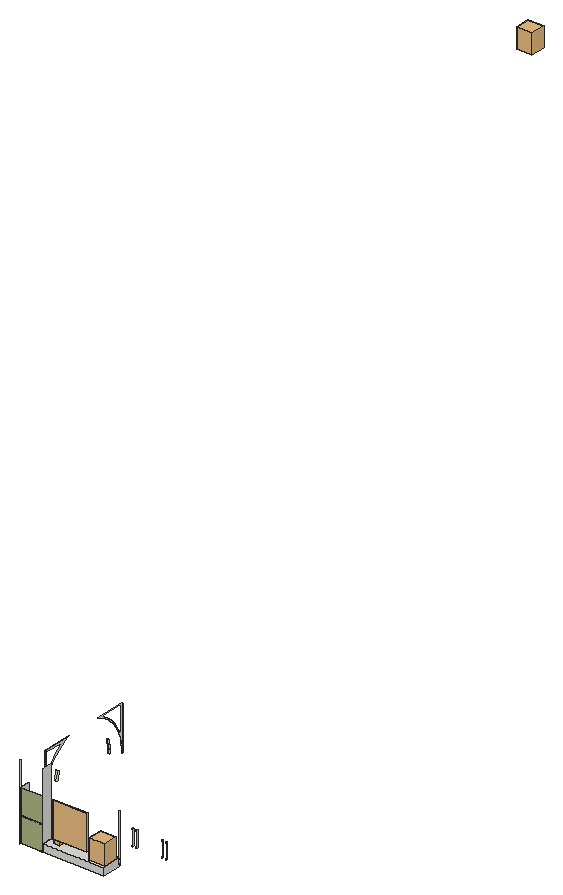
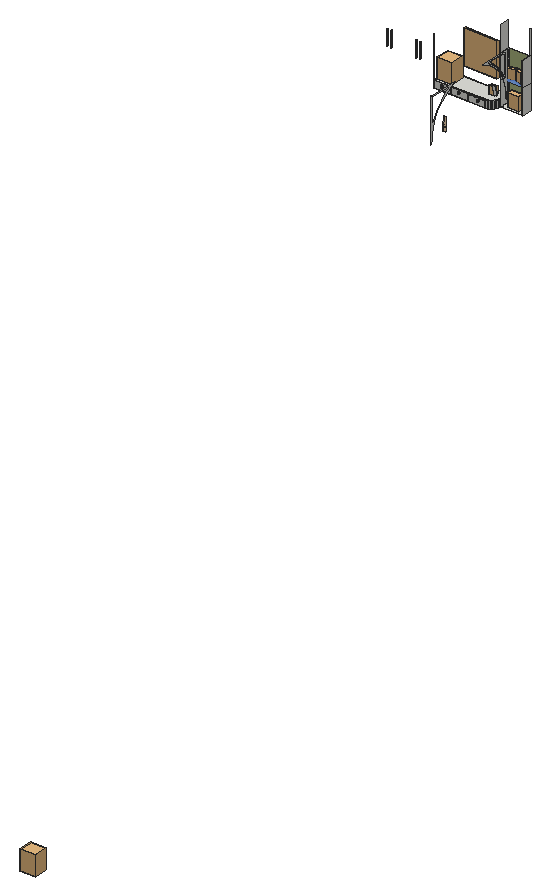
# SketchUp Ruby script. Lengths in inches.
U = 1.inch
M = Sketchup.active_model
def pt(a) = Geom::Point3d.new(a.map { |v| v * U })
def face(e, loops, mat)
  f = e.add_face(loops[0].map { |a| pt(a) })
  loops[1..].each { |l| e.add_face(l.map { |a| pt(a) }).erase! }
  f.material = f.back_material = mat if mat
  f
end
# faces: each face lists its corners as indices into pts; further lists are holes
def faces(e, pts, list, mat = nil) = list.each { |f| face(e, (f[0].is_a?(Array) ? f : [f]).map { |l| l.map { |i| pts[i] } }, mat) }
# xy, xz, yz: faces in a plane at the given z, y or x. An outline is a flat list of corners, or four numbers for a rectangle; further outlines are holes
def ring(l) = l.size == 4 ? [[l[0], l[1]], [l[2], l[1]], [l[2], l[3]], [l[0], l[3]]] : l.each_slice(2).to_a
def flat(e, list, mat, &to3) = list.each { |f| face(e, (f[0].is_a?(Array) ? f : [f]).map { |l| ring(l).map { |u, v| to3.(u, v) } }, mat) }
def xy(e, z, list, mat = nil) = flat(e, list, mat) { |x, y| [x, y, z] }
def xz(e, y, list, mat = nil) = flat(e, list, mat) { |x, z| [x, y, z] }
def yz(e, x, list, mat = nil) = flat(e, list, mat) { |y, z| [x, y, z] }
def lines(e, pts, list) = list.each { |a, b| e.add_line(pt(pts[a]), pt(pts[b])) }
# prism: a flat outline (further loops are holes) pulled along v
def prism(e, loops, v, mat = nil)
  f = face(e, loops, mat); d = Geom::Vector3d.new(v.map { |x| x * U })
  f.pushpull(f.normal.samedirection?(d) ? d.length : -d.length)
end
def box(e, o, s, mat = nil) = prism(e, [[o, [o[0] + s[0], o[1], o[2]], [o[0] + s[0], o[1] + s[1], o[2]], [o[0], o[1] + s[1], o[2]]]], [0, 0, s[2]], mat)
def at(x, y, z, deg = 0) = Geom::Transformation.translation(pt([x, y, z])) * Geom::Transformation.rotation(ORIGIN, Z_AXIS, deg.degrees)
def axes(o, x, y, z) = Geom::Transformation.new([*x, 0, *y, 0, *z, 0, *pt(o).to_a, 1])
def part(name) = M.definitions.add(name)
# library, detail: a bought-in or finely detailed component or shape, given as its bounding box
def library(name, o, s) = part(name).tap { |d| box(d.entities, o, s) }
def detail(e, o, s) = box(e.add_group.entities, o, s)
def put(e, d, t, mat = nil) = e.add_instance(d, t).tap { |i| i.material = mat if mat }
def group(e, t, mat = nil) = e.add_group.tap { |g| g.transformation = t; g.material = mat if mat }.entities
root = M.entities
M.materials.add("Emissive").color = [255, 225, 187]
M.materials.add("[Translucent Glass Blue]").color = [100, 149, 237]
M.materials["[Translucent Glass Blue]"].alpha = 0.5
M.materials.add("cubod").color = [174, 185, 130]
c1 = library("POTICHES",[0,0,0],[13.49,6.56,16.28])
c2 = part("Group\#11")
xz(c2.entities,1.09,[[1.15,0,0.85,0.04,0.57,0.15,0.34,0.33,0.15,0.56,0.04,0.83,0,1.12,0.04,1.41,0.15,1.68,0.34,1.91,0.57,2.09,0.85,2.2,1.15,2.24,1.45,2.2,1.72,2.09,1.96,1.91,2.14,1.68,2.26,1.41,2.3,1.12,2.26,0.83,2.14,0.56,1.96,0.33,1.72,0.15,1.45,0.04]])
p = [[0.57,1.09,0.15],[0.85,1.09,0.04],[0.85,0.7,0.04],[0.57,0.7,0.15],[1.15,1.09,0],[1.15,0.7,0],
  [1.45,1.09,0.04],[1.45,0.7,0.04],[1.72,1.09,0.15],[1.72,0.7,0.15],[0.34,1.09,0.33],[0.34,0.7,0.33],
  [1.96,1.09,0.33],[1.96,0.7,0.33],[0.15,1.09,0.56],[0.15,0.7,0.56],[2.14,1.09,0.56],[2.14,0.7,0.56],
  [1.02,0.7,0.65],[1.15,0.7,0.64],[1.15,0,0.64],[1.02,0,0.65],[1.28,0.7,0.65],[1.28,0,0.65],
  [0.04,1.09,0.83],[0.04,0.7,0.83],[2.26,1.09,0.83],[2.26,0.7,0.83],[0.8,0.7,0.78],[0.9,0.7,0.7],
  [0.9,0,0.7],[0.8,0,0.78],[1.4,0.7,0.7],[1.4,0,0.7],[1.5,0.7,0.78],[1.5,0,0.78],
  [0.72,0.7,0.88],[0.72,0,0.88],[1.58,0.7,0.88],[1.58,0,0.88],[0,1.09,1.12],[0,0.7,1.12],
  [2.3,1.09,1.12],[2.3,0.7,1.12],[0.67,0.7,0.99],[0.67,0,0.99],[1.63,0.7,0.99],[1.63,0,0.99],
  [0.65,0.7,1.12],[0.65,0,1.12],[1.65,0.7,1.12],[1.65,0,1.12],[0.67,0.7,1.25],[0.67,0,1.25],
  [1.63,0.7,1.25],[1.63,0,1.25],[0.04,1.09,1.41],[0.04,0.7,1.41],[2.26,1.09,1.41],[2.26,0.7,1.41],
  [0.72,0.7,1.36],[0.72,0,1.36],[1.58,0.7,1.36],[1.58,0,1.36],[0.8,0.7,1.46],[0.8,0,1.46],
  [1.5,0.7,1.46],[1.5,0,1.46],[0.15,1.09,1.68],[0.15,0.7,1.68],[2.14,1.09,1.68],[2.14,0.7,1.68],
  [0.9,0.7,1.54],[0.9,0,1.54],[1.02,0.7,1.59],[1.02,0,1.59],[1.4,0.7,1.54],[1.28,0.7,1.59],
  [1.28,0,1.59],[1.4,0,1.54],[1.15,0.7,1.6],[1.15,0,1.6],[0.34,1.09,1.91],[0.34,0.7,1.91],
  [1.96,1.09,1.91],[1.96,0.7,1.91],[0.57,1.09,2.09],[0.57,0.7,2.09],[1.72,1.09,2.09],[1.72,0.7,2.09],
  [0.85,1.09,2.2],[0.85,0.7,2.2],[1.45,1.09,2.2],[1.45,0.7,2.2],[1.15,1.09,2.24],[1.15,0.7,2.24]]
faces(c2.entities,p,[[0,1,2,3],[1,4,5,2],[4,6,7,5],[6,8,9,7],[10,0,3,11],[8,12,13,9],[14,10,11,15],[12,16,17,13],
  [18,19,20,21],[19,22,23,20],[24,14,15,25],[16,26,27,17],[28,29,30,31],[29,18,21,30],[22,32,33,23],[32,34,35,33],
  [36,28,31,37],[34,38,39,35],[40,24,25,41],[26,42,43,27],[44,36,37,45],[38,46,47,39],[48,44,45,49],[46,50,51,47],
  [52,48,49,53],[50,54,55,51],[56,40,41,57],[42,58,59,43],[60,52,53,61],[54,62,63,55],[64,60,61,65],[62,66,67,63],
  [68,56,57,69],[58,70,71,59],[72,64,65,73],[74,72,73,75],[76,77,78,79],[66,76,79,67],[80,74,75,81],[77,80,81,78],
  [82,68,69,83],[70,84,85,71],[86,82,83,87],[84,88,89,85],[90,86,87,91],[88,92,93,89],[94,90,91,95],[92,94,95,93]])
c3 = library("Vase with branches",[15.48,-1.66,0],[18.51,16.76,23.67])
c4 = library("Decor Livro e Telescópio",[-0.65,0.19,2.02],[7.35,4.61,9.12])
c5 = part("Group\#10")
prism(c5.entities,[[[1.125,0,43.59],[1.125,0,42.2],[1.125,4.02,42.2],[1.125,4.02,1.84],[1.125,3.28,1.84],[1.125,0,1.84],[1.125,0,0],[1.125,4.41,0],[1.125,4.53,0.01],[1.125,4.64,0.03],[1.125,4.76,0.07],[1.125,4.86,0.12],[1.125,4.96,0.1875],[1.125,5.05,0.26],[1.125,5.125,0.35],[1.125,5.19,0.45],[1.125,5.24,0.56],[1.125,5.28,0.67],[1.125,5.3,0.79],[1.125,5.3125,0.9],[1.125,5.3125,42.39],[1.125,5.3,42.54],[1.125,5.28,42.68],[1.125,5.23,42.82],[1.125,5.17,42.95],[1.125,5.1,43.08],[1.125,5,43.19],[1.125,4.9,43.3],[1.125,4.78,43.39],[1.125,4.66,43.46],[1.125,4.52,43.52],[1.125,4.38,43.56],[1.125,4.24,43.59]]],[-0.5625,0,0])
c6 = library("Agrupar\#9",[-3.82,0,-0.04],[36.26,88.57,114.21])
c7 = library("Agrupar\#8",[-3.82,0,-0.04],[36.26,88.57,114.21])
xy(root,34.31,[[616.04,4,616.04,16,616.12,17.36,616.35,18.7,616.73,20.01,617.25,21.26,617.92,22.45,618.71,23.56,619.63,24.5625,620.65,25.46,621.77,26.24,622.97,26.88,623.25,27,688.79,27,688.79,4]])
xy(root,34.39,[[589.4375,4,613.52,4.375],[613.52,4,615.39,4.375],[589.4375,4.375,615.39,16]])
xy(root,34.81,[[623.25,27,624.23,27.39,625.54,27.75,646.47,27.75,646.47,27.0625,646.625,27.0625,646.625,27.75,667.55,27.75,667.55,27.0625,667.71,27.0625,667.71,27.75,688.79,27.75,688.79,27]])
xy(root,42.88,[[623.25,27,688.79,27,688.79,27.75,667.71,27.75,667.71,27.0625,667.55,27.0625,667.55,27.75,646.625,27.75,646.625,27.0625,646.47,27.0625,646.47,27.75,625.54,27.75,624.23,27.39]])
xy(root,43.44,[[616.04,4,688.79,4,688.79,27,623.25,27,622.97,26.88,621.77,26.24,620.65,25.46,619.63,24.5625,618.71,23.56,617.92,22.45,617.25,21.26,616.73,20.01,616.35,18.7,616.12,17.36,616.04,16]])
xy(root,64,[[589.4375,4,613.52,4.375],[613.52,4,615.39,4.375]])
xy(root,64,[[589.4375,4.375,615.39,16]],"[Translucent Glass Blue]")
xy(root,64.39,[[589.4375,4,615.39,4.375]])
xy(root,64.39,[[589.4375,4.375,615.39,16]],"[Translucent Glass Blue]")
xz(root,4,[[616.04,34.31,688.79,43.44],[614.17,34.38,615.39,34.38,615.39,34.39,613.52,34.39],[615.39,34.39,616.04,94.39],[588.79,64,589.4375,124],[589.4375,64,615.39,64.39]])
xz(root,4.375,[[589.4375,34.39,615.39,64],[589.4375,64.39,615.39,94]],"cubod")
xz(root,16,[[614.17,34.38,613.52,34.39,615.39,34.39,615.39,34.38]])
xz(root,27,[[623.25,34.31,688.79,34.81],[623.25,42.88,688.79,43.44]])
xz(root,27.0625,[[646.47,34.81,646.625,42.88],[667.55,34.81,667.71,42.88]])
xz(root,27.75,[[[625.54,34.81,646.47,42.88],[634,39.6,634.13,39.62,634.25,39.67,634.35,39.75,634.43,39.85,634.48,39.96,634.5,40.09,634.48,40.21,634.43,40.33,634.35,40.43,634.25,40.51,634.13,40.56,634,40.57,633.875,40.56,633.75,40.51,633.65,40.43,633.57,40.33,633.52,40.21,633.5,40.09,633.52,39.96,633.57,39.85,633.65,39.75,633.75,39.67,633.875,39.62]],[646.625,34.81,667.55,42.88],[667.71,34.81,688.79,42.88],[634,39.6,633.875,39.62,633.75,39.67,633.65,39.75,633.57,39.85,633.52,39.96,633.5,40.09,633.52,40.21,633.57,40.33,633.65,40.43,633.75,40.51,633.875,40.56,634,40.57,634.13,40.56,634.25,40.51,634.35,40.43,634.43,40.33,634.48,40.21,634.5,40.09,634.48,39.96,634.43,39.85,634.35,39.75,634.25,39.67,634.13,39.62]])
xz(root,28.45,[[[634,38.97,634.3,39.01,634.58,39.12,634.8125,39.3,635,39.53,635.11,39.8,635.15,40.09,635.11,40.38,635,40.65,634.8125,40.88,634.58,41.06,634.3,41.17,634,41.21,633.7,41.17,633.43,41.06,633.1875,40.88,633.01,40.65,632.89,40.38,632.85,40.09,632.89,39.8,633.01,39.53,633.1875,39.3,633.43,39.12,633.7,39.01],[634,39.6,633.875,39.62,633.75,39.67,633.65,39.75,633.57,39.85,633.52,39.96,633.5,40.09,633.52,40.21,633.57,40.33,633.65,40.43,633.75,40.51,633.875,40.56,634,40.57,634.13,40.56,634.25,40.51,634.35,40.43,634.43,40.33,634.48,40.21,634.5,40.09,634.48,39.96,634.43,39.85,634.35,39.75,634.25,39.67,634.13,39.62]]])
xz(root,41.03,[[588.45,64,588.79,117.17]])
xz(root,41.03,[[588.1,64,588.45,117.17]],"Emissive")
xz(root,41.82,[[588.1,77.21,588.79,116.375]],"Emissive")
xz(root,138.88,[[587.07,71.16,588.79,76.51]])
xz(root,138.88,[[585.35,71.16,587.07,76.51]],"Emissive")
xz(root,157.17,[[588.45,64,588.79,117.17]])
xz(root,157.17,[[588.1,64,588.45,117.17]],"Emissive")
yz(root,588.1,[[[41.03,64,41.3,69.59,42.12,75.12,43.48,80.54,45.36,85.81,47.74,90.87,50.61,95.67,53.94,100.16,57.69,104.3125,61.83,108.07,66.32,111.41,71.11,114.29,76.16,116.7,77.31,117.17,41.03,117.17],[41.82,77.21,41.82,116.375,73.63,116.375,70.73,115,65.875,112.07,61.32,108.6875,57.13,104.875,53.33,100.67,49.95,96.11,47.04,91.24,44.62,86.11,42.71,80.77]],[[157.17,64,157.17,117.17,121.42,117.17,122.57,116.7,127.65,114.37,132.47,111.53,136.98,108.22,141.13,104.47,144.87,100.31,148.18,95.8,151,90.98,153.33,85.89,155.12,80.59,156.37,75.14,157.05,69.59],[156.375,78.67,155.89,80.81,154.07,86.18,151.71,91.34,148.84,96.24,145.49,100.82,141.69,105.03,137.48,108.84,132.91,112.2,128.02,115.07,125.18,116.375,156.375,116.375]]])
yz(root,588.79,[[4,34,16,64],[4,64,16,94],[[41.82,77.21,42.71,80.77,44.62,86.11,47.04,91.24,49.95,96.11,53.33,100.67,57.13,104.875,61.32,108.6875,65.875,112.07,70.73,115,73.63,116.375,41.82,116.375],[43.01,85.13,43.01,115.1875,68.75,115.1875,65.21,113.06,60.57,109.6,56.29,105.71,52.41,101.42,48.96,96.77,45.99,91.8,43.52,86.57]]])
yz(root,589.4375,[[4,34.39,4.375,64],[4.375,34.39,16,64],[4,64.39,4.375,94],[4.375,64.39,16,94]])
yz(root,615.39,[[4,33.99,16,34],[4,34.38,16,34.39],[4,34.39,4.375,64],[4.375,34.39,16,64],[4,64.39,4.375,94],
  [4.375,64.39,16,94]])
yz(root,616.04,[[4,34.31,16,43.44],[4,43.44,16,124]])
yz(root,646.47,[[27.0625,34.81,27.75,42.88]])
yz(root,646.625,[[27.0625,34.81,27.75,42.88]])
yz(root,667.55,[[27.0625,34.81,27.75,42.88]])
yz(root,667.71,[[27.0625,34.81,27.75,42.88]])
yz(root,688.79,[[4,34.31,27,43.44],[27,34.81,27.75,36.56],[27,36.56,27.75,37.05],[27,37.05,27.75,37.36],[27,37.36,27.75,42.88],
  [27,42.88,27.75,93.69]])
p = [[616.04,16,43.44],[616.12,17.36,43.44],[616.12,17.36,34.31],[616.04,16,34.31],[616.35,18.7,43.44],[616.35,18.7,34.31],
  [616.73,20.01,43.44],[616.73,20.01,34.31],[617.25,21.26,43.44],[617.25,21.26,34.31],[617.92,22.45,43.44],[617.92,22.45,34.31],
  [618.71,23.56,43.44],[618.71,23.56,34.31],[619.63,24.5625,43.44],[619.63,24.5625,34.31],[620.65,25.46,43.44],[620.65,25.46,34.31],
  [621.77,26.24,43.44],[621.77,26.24,34.31],[622.97,26.88,43.44],[622.97,26.88,34.31],[623.25,27,43.44],[623.25,27,42.88],
  [623.25,27,34.81],[623.25,27,34.31],[624.23,27.39,42.88],[624.23,27.39,34.81],[625.54,27.75,42.88],[625.54,27.75,34.81],
  [588.1,41.03,64],[588.45,41.03,64],[588.45,41.3,69.59],[588.1,41.3,69.59],[588.79,41.3,69.59],[588.79,41.03,64],
  [588.1,157.05,69.59],[588.45,157.05,69.59],[588.45,157.17,64],[588.1,157.17,64],[588.79,157.17,64],[588.79,157.05,69.59],
  [588.45,42.12,75.12],[588.1,42.12,75.12],[588.79,42.12,75.12],[588.1,156.37,75.14],[588.45,156.37,75.14],[588.79,156.37,75.14],
  [588.45,43.48,80.54],[588.1,43.48,80.54],[588.79,43.48,80.54],[588.1,155.12,80.59],[588.45,155.12,80.59],[588.79,155.12,80.59],
  [585.35,61.19,86.73],[587.07,61.19,86.73],[587.07,59.84,76.51],[585.35,59.84,76.51],[588.79,59.84,76.51],[588.79,61.19,86.73],
  [585.35,138.88,76.51],[587.07,138.88,76.51],[587.07,137.54,86.73],[585.35,137.54,86.73],[588.79,137.54,86.73],[588.79,138.88,76.51],
  [588.79,42.71,80.77],[588.79,41.82,77.21],[588.1,41.82,77.21],[588.1,42.71,80.77],[615.39,16,34.38],[615.39,16,34],
  [589.4375,16,34.39],[589.4375,16,34]]
faces(root,p,[[0,1,2,3],[1,4,5,2],[4,6,7,5],[6,8,9,7],[8,10,11,9],[10,12,13,11],[12,14,15,13],[14,16,17,15],
  [16,18,19,17],[18,20,21,19],[20,22,23,24,25,21],[24,23,26,27],[27,26,28,29],[34,32,31,35],[40,38,37,41],[44,42,32,34],
  [41,37,46,47],[50,48,42,44],[47,46,52,53],[58,56,55,59],[64,62,61,65]])
faces(root,p,[[30,31,32,33],[36,37,38,39],[33,32,42,43],[45,46,37,36],[43,42,48,49],[51,52,46,45],[54,55,56,57],[60,61,62,63],
  [66,67,68,69]],"Emissive")
lines(root,p,[[70,71],[72,73]])
put(root,c1,at(609.77,12.93,34.39,180))
put(root,c2,at(632.85,27.75,38.97))
put(root,c2,at(656.23,27.75,38.97))
put(root,c2,at(677.1,27.75,38.97))
put(root,c3,at(46.95,1483.23,42.65,180))
put(root,c4,at(629.89,15.98,41.42,180))
put(root,c3,at(703,22.14,43.44,180))
g1 = group(root,at(629.8,2.375,55.04))
detail(g1,[0,-1.0625,0],[40.89,2.3,40.89])
put(root,c5,axes([703.5,27.75,61],[1,0,0],[0,0.20009,0],[0,0,0.4371]))
put(root,c5,axes([708.375,27.75,61],[1,0,0],[0,0.20009,0],[0,0,0.4371]))
put(root,c5,axes([744.1875,27.75,61],[1,0,0],[0,0.20009,0],[0,0,0.4371]))
put(root,c5,axes([739.3125,27.75,61],[1,0,0],[0,0.20009,0],[0,0,0.4371]))
put(root,c6,axes([592.25,9.25,64.39],[0.03072,0.10437,0],[0.10437,-0.03072,0],[0,0,0.1088]))
put(root,c7,axes([612.74,9.25,64.39],[-0.03072,0.10437,0],[-0.10437,-0.03072,0],[0,0,0.1088]))
